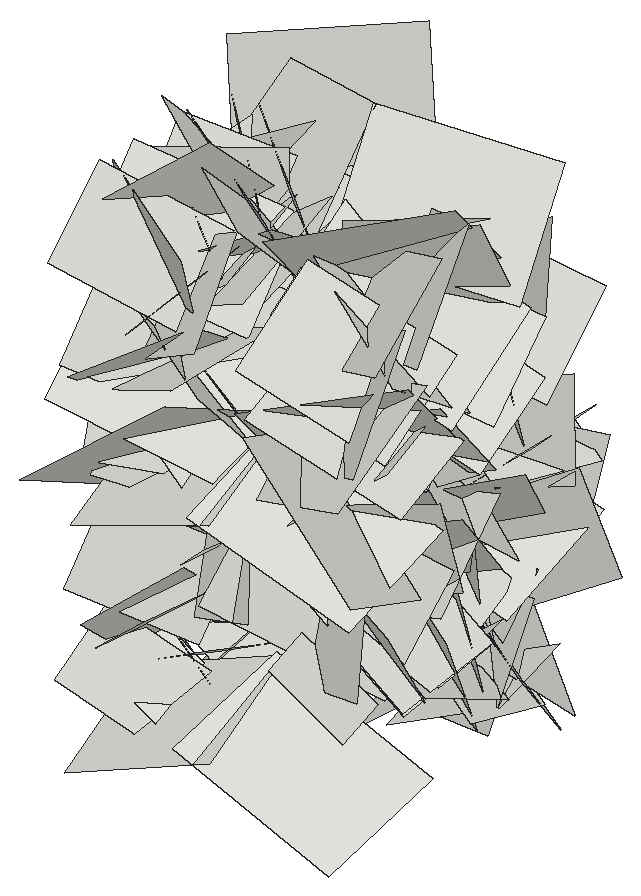
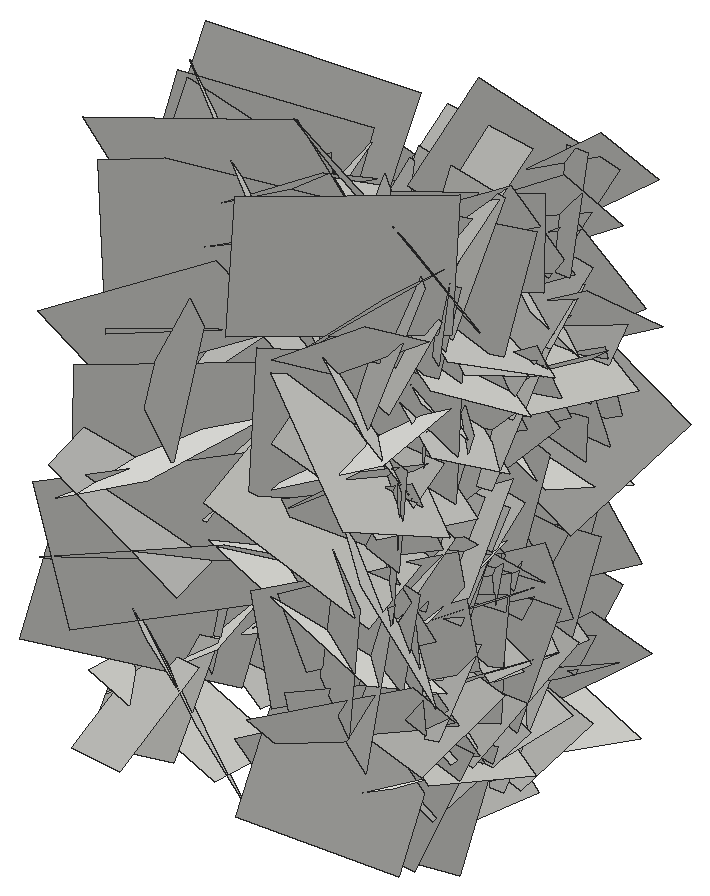
# SketchUp Ruby script. Lengths in inches.
U = 1.inch
M = Sketchup.active_model
def pt(a) = Geom::Point3d.new(a.map { |v| v * U })
def face(e, loops, mat)
  f = e.add_face(loops[0].map { |a| pt(a) })
  loops[1..].each { |l| e.add_face(l.map { |a| pt(a) }).erase! }
  f.material = f.back_material = mat if mat
  f
end
# faces: each face lists its corners as indices into pts; further lists are holes
def faces(e, pts, list, mat = nil) = list.each { |f| face(e, (f[0].is_a?(Array) ? f : [f]).map { |l| l.map { |i| pts[i] } }, mat) }
# xy, xz, yz: faces in a plane at the given z, y or x. An outline is a flat list of corners, or four numbers for a rectangle; further outlines are holes
def ring(l) = l.size == 4 ? [[l[0], l[1]], [l[2], l[1]], [l[2], l[3]], [l[0], l[3]]] : l.each_slice(2).to_a
def flat(e, list, mat, &to3) = list.each { |f| face(e, (f[0].is_a?(Array) ? f : [f]).map { |l| ring(l).map { |u, v| to3.(u, v) } }, mat) }
def xy(e, z, list, mat = nil) = flat(e, list, mat) { |x, y| [x, y, z] }
def xz(e, y, list, mat = nil) = flat(e, list, mat) { |x, z| [x, y, z] }
def yz(e, x, list, mat = nil) = flat(e, list, mat) { |y, z| [x, y, z] }
def lines(e, pts, list) = list.each { |a, b| e.add_line(pt(pts[a]), pt(pts[b])) }
# prism: a flat outline (further loops are holes) pulled along v
def prism(e, loops, v, mat = nil)
  f = face(e, loops, mat); d = Geom::Vector3d.new(v.map { |x| x * U })
  f.pushpull(f.normal.samedirection?(d) ? d.length : -d.length)
end
def box(e, o, s, mat = nil) = prism(e, [[o, [o[0] + s[0], o[1], o[2]], [o[0] + s[0], o[1] + s[1], o[2]], [o[0], o[1] + s[1], o[2]]]], [0, 0, s[2]], mat)
def at(x, y, z, deg = 0) = Geom::Transformation.translation(pt([x, y, z])) * Geom::Transformation.rotation(ORIGIN, Z_AXIS, deg.degrees)
def axes(o, x, y, z) = Geom::Transformation.new([*x, 0, *y, 0, *z, 0, *pt(o).to_a, 1])
def part(name) = M.definitions.add(name)
# library, detail: a bought-in or finely detailed component or shape, given as its bounding box
def library(name, o, s) = part(name).tap { |d| box(d.entities, o, s) }
def detail(e, o, s) = box(e.add_group.entities, o, s)
def put(e, d, t, mat = nil) = e.add_instance(d, t).tap { |i| i.material = mat if mat }
def group(e, t, mat = nil) = e.add_group.tap { |g| g.transformation = t; g.material = mat if mat }.entities
root = M.entities
c1 = part("Component\#6")
p = [[0.01,0,0],[0,3.24,4.54],[4.32,3.24,4.54],[4.33,0,0]]
faces(c1.entities,p,[[0,1,2,3]])
put(root,c1,axes([414.68,163.43,17.5],[0.07736,-0.30856,0.98844],[0.18729,0.98007,0.2929],[-1.08152,0.14765,0.12143]))
put(root,c1,axes([410.71,163.43,17.5],[-0.07736,-0.30856,0.98844],[-0.18729,0.98007,0.2929],[1.08152,0.14765,0.12143]))
put(root,c1,axes([410.71,155.625,2.89],[0.13104,0.56412,0.5606],[-0.11872,0.57403,-0.55293],[0.83462,-0.00692,-0.16667]))
put(root,c1,axes([410.71,168.54,15.47],[-0.051,0.16682,-0.79913],[0.09039,-0.79511,-0.17112],[0.86061,0.0934,-0.02938]))
put(root,c1,axes([414.68,164.44,22.83],[0.02931,-0.02413,-0.88007],[0.04764,-0.87932,0.02552],[-0.93201,-0.0457,-0.02637]))
put(root,c1,axes([410.71,159.9,13.67],[-0.02397,0.44215,0.82689],[-0.11898,0.8199,-0.44149],[0.98679,0.1096,-0.03314]))
put(root,c1,axes([410.71,159.79,6],[-0.13547,0.51146,0.93772],[-0.15367,0.92736,-0.52557],[1.12174,0.18881,0.04125]))
put(root,c1,axes([414.68,165.07,9.38],[-0.13081,0.27606,-0.70722],[0.08788,-0.70731,-0.29057],[-0.79993,-0.12284,0.08373]))
put(root,c1,axes([410.71,167.39,19.82],[0.12929,0.6108,0.35138],[0.02449,0.35295,-0.62154],[0.74654,-0.11736,-0.04046]))
put(root,c1,axes([410.71,155.24,20.59],[0.01301,0.69003,0.71111],[-0.211,0.69839,-0.67424],[1.02891,0.13449,-0.14726]))
put(root,c1,axes([410.71,164.66,7.18],[-0.03191,0.54978,-0.59147],[0.106,-0.58478,-0.54866],[0.84939,0.09364,0.04625]))
put(root,c1,axes([410.71,167.84,10.46],[-0.01526,0.23241,-0.73689],[0.14958,-0.72384,-0.23105],[0.80526,0.13886,0.02896]))
put(root,c1,axes([410.71,166.25,3.34],[0.10377,-0.78092,-0.09398],[-0.04515,-0.09983,0.78516],[0.83253,0.09192,0.05429]))
put(root,c1,axes([410.71,166.67,11.65],[0.03639,0.32382,0.70516],[0.0632,0.70266,-0.32558],[0.82009,-0.06852,-0.0062]))
put(root,c1,axes([414.68,164.7,6.68],[0.19863,-0.78204,0.62344],[0.03401,0.63866,0.7915],[-1.0596,-0.1261,0.14227]))
put(root,c1,axes([414.68,165.06,16.01],[0.24936,0.99659,0.4051],[0.07669,0.39908,-1.02378],[-1.13774,0.24532,0.01978]))
put(root,c1,axes([414.68,162.4,12.14],[-0.15913,-0.1111,0.71617],[0.10617,0.72117,0.13287],[-0.76084,0.12387,-0.13124]))
put(root,c1,axes([410.71,166.02,4.84],[-0.16866,0.71959,0.68076],[0.0323,0.69272,-0.72511],[1.04952,0.09433,0.13172]))
put(root,c1,axes([410.71,157.37,3.29],[0.12325,0.67494,0.21472],[0.06797,0.20667,-0.68436],[0.74769,-0.13004,0.02682]))
put(root,c1,axes([410.71,162.54,0.74],[-0.05881,-0.79857,0.25436],[0.14334,0.24305,0.79255],[0.87675,-0.0933,-0.11251]))
put(root,c1,axes([410.71,164.04,2.37],[-0.08884,-0.86849,0.07962],[0.14736,0.06566,0.86256],[0.91264,-0.09515,-0.13152]))
put(root,c1,axes([414.68,167.12,21.5],[-0.0656,0.35319,-0.61189],[-0.00255,-0.61434,-0.35436],[-0.7489,-0.02885,0.0548]))
put(root,c1,axes([414.68,165.55,15.88],[0.02597,-0.35934,-0.67832],[-0.02345,-0.67872,0.35875],[-0.81334,0.00809,-0.032]))
put(root,c1,axes([414.68,169.26,18.83],[-0.02849,-0.83115,-0.05333],[0.13283,-0.05679,0.82186],[-0.87278,0.01849,0.12683]))
put(root,c1,axes([410.71,168.08,9.41],[-0.11593,0.02752,-0.90523],[0.14705,-0.90054,-0.04413],[0.94866,0.14295,-0.10378]))
put(root,c1,axes([414.68,161.46,7.67],[-0.11157,-0.00104,0.59962],[-0.09459,0.60203,-0.01462],[-0.62852,-0.09042,-0.10424]))
put(root,c1,axes([414.68,169.83,13.22],[-0.13817,-0.64015,-0.16037],[0.03989,-0.17041,0.64965],[-0.69839,0.11692,0.06883]))
put(root,c1,axes([410.71,170.98,12.21],[-0.31631,-0.51758,-1.19288],[-0.16648,-1.20059,0.56021],[1.36826,-0.26573,-0.20761]))
put(root,c1,axes([414.68,164.04,15.7],[-0.03624,-0.6234,-0.24842],[-0.08,-0.24359,0.62167],[-0.70683,0.05954,-0.05762]))
put(root,c1,axes([414.68,160.57,3.12],[-0.03509,0.82869,0.13415],[0.15764,0.13792,-0.81528],[-0.87577,-0.00838,-0.15213]))
put(root,c1,axes([410.71,159.03,23.29],[-0.13252,0.38295,-0.87838],[0.10893,-0.87536,-0.39626],[1.00987,0.14467,-0.07253]))
put(root,c1,axes([414.68,166.8,6.58],[0.19077,-0.84984,-0.315],[-0.00737,-0.32244,0.86593],[-0.9607,-0.16629,-0.0692]))
put(root,c1,axes([410.71,166.22,16.78],[-0.0558,0.90138,-0.08554],[0.09664,-0.07998,-0.89882],[0.95488,0.06076,0.08597]))
put(root,c1,axes([414.68,159.32,12.84],[-0.06752,-0.16321,-0.59207],[-0.0871,-0.58763,0.17083],[-0.64514,0.09641,0.0389]))
put(root,c1,axes([410.71,167.39,3.05],[-0.22625,-1.02118,-0.283],[0.12014,-0.30902,1.02962],[1.11681,-0.17363,-0.16809]))
put(root,c1,axes([414.68,159.79,25.07],[0.1328,0.69586,-0.68383],[0.18687,-0.69425,-0.67416],[-1.01714,-0.03669,-0.21313]))
put(root,c1,axes([410.71,163.26,10.51],[0.09772,0.8385,-0.3881],[-0.10419,-0.37892,-0.842],[0.97385,-0.12468,-0.05114]))
put(root,c1,axes([414.68,160.97,6.7],[-0.04912,0.73058,0.10133],[0.09877,0.10652,-0.72536],[-0.77557,-0.03271,-0.0988]))
put(root,c1,axes([410.71,170.16,13.55],[-0.14984,-1.04824,-0.22204],[0.00627,-0.22472,1.05715],[1.13577,-0.13705,-0.03513]))
put(root,c1,axes([414.68,161.26,10.83],[0.08958,0.45503,-0.59155],[-0.06652,-0.58889,-0.46195],[-0.78829,0.10141,-0.02824]))
put(root,c1,axes([414.68,160.54,14.42],[0.065,-0.29459,-0.75204],[0.0763,-0.74921,0.29935],[-0.85274,-0.0895,-0.03054]))
put(root,c1,axes([414.68,160.65,18.69],[-0.1336,-0.1743,0.59472],[0.06624,0.60023,0.18916],[-0.65357,0.09646,-0.1024]))
put(root,c1,axes([414.68,159.61,12.59],[-0.0897,0.16152,-0.57424],[-0.01993,-0.58042,-0.16049],[-0.632,-0.00462,0.08656]))
put(root,c1,axes([410.71,169.09,13.37],[0.12805,-0.81492,0.2825],[-0.01832,0.28292,0.8235],[0.91406,0.11983,-0.02307]))
put(root,c1,axes([414.68,158.82,19.64],[-0.09205,0.73549,-0.019],[0.17536,0.00088,-0.72213],[-0.75991,-0.08889,-0.16434]))
put(root,c1,axes([410.71,166.72,20.27],[0.14718,0.45385,-0.66356],[0.05291,-0.67695,-0.45256],[0.85051,-0.03642,0.14299]))
put(root,c1,axes([410.71,158.84,13.7],[0.15038,-0.75335,0.50607],[-0.08727,0.49942,0.76653],[0.95804,0.16374,-0.00961]))
put(root,c1,axes([410.71,161.03,4.22],[0.00206,0.54706,-0.73945],[0.10036,-0.73565,-0.544],[0.96983,0.07497,0.05787]))
put(root,c1,axes([410.71,167.74,3.51],[-0.11337,-0.86322,0.3774],[0.28126,0.33685,0.84566],[0.95821,-0.201,-0.20357]))
put(root,c1,axes([410.71,165.75,-1.09],[-0.03685,-0.4153,0.96157],[-0.02645,0.96216,0.41465],[1.10996,0.00914,0.04181]))
put(root,c1,axes([410.71,165.51,17.74],[0.00528,-0.97827,-0.44464],[-0.11526,-0.44282,0.97306],[1.13321,-0.04048,0.10104]))
put(root,c1,axes([414.68,158.25,7.85],[-0.01053,0.60228,-0.51533],[0.19634,-0.49934,-0.58716],[-0.81696,-0.12777,-0.13447]))
put(root,c1,axes([414.68,167.39,12.19],[0.06725,0.11282,-0.6237],[-0.12717,-0.61335,-0.12315],[-0.65971,0.12973,-0.03984]))
put(root,c1,axes([414.68,164.71,11.17],[0.09162,-0.23701,0.75882],[0.09076,0.76162,0.22813],[-0.83777,0.05659,0.1077]))
put(root,c1,axes([410.71,164.72,6.23],[-0.02586,0.29335,1.1723],[-0.23754,1.1511,-0.29271],[1.25874,0.22326,-0.03115]))
put(root,c1,axes([414.68,159.82,10.86],[0.164,0.05549,-0.7166],[-0.119,-0.72215,-0.08015],[-0.75252,0.12629,-0.14349]))
put(root,c1,axes([410.71,167.01,8.33],[0.18631,0.3359,0.73427],[0.04897,0.74605,-0.35235],[0.8545,-0.11599,-0.1399]))
put(root,c1,axes([410.71,166.18,19.56],[-0.12535,0.0531,1.28965],[-0.2192,1.27754,-0.07157],[1.35051,0.21229,0.10808]))
put(root,c1,axes([410.71,168.14,0.12],[-0.06773,-0.63363,0.78179],[0.11595,0.77435,0.63654],[1.06038,-0.12515,-0.01967]))
put(root,c1,axes([410.71,169.19,10.7],[-0.0913,0.46499,-1.24639],[-0.29576,-1.22753,-0.43867],[1.37875,-0.23253,-0.17663]))
put(root,c1,axes([414.68,165.96,10.85],[0.09912,0.20412,-0.70693],[0.02587,-0.71308,-0.20267],[-0.77953,0.00229,-0.09661]))
put(root,c1,axes([414.68,161.25,17.66],[0.25985,0.898,-0.37026],[0.14737,-0.41038,-0.90325],[-1.01902,0.16964,-0.22504]))
put(root,c1,axes([414.68,162.79,15.86],[0.07285,0.46729,0.4905],[-0.02436,0.49435,-0.46773],[-0.71769,0.03066,0.06566]))
put(root,c1,axes([410.71,167.22,15.375],[-0.0235,-0.92066,-0.53568],[-0.01768,-0.53543,0.92093],[1.12894,-0.02755,0.00327]))
put(root,c1,axes([410.71,167.28,17.92],[-0.19972,-0.96368,-0.57877],[0.14667,-0.60226,0.95775],[1.18251,-0.08806,-0.21655]))
put(root,c1,axes([410.71,157.18,19.73],[-0.07599,0.81527,0.8297],[-0.084,0.82592,-0.8184],[1.23014,0.10676,-0.00463]))
put(root,c1,axes([410.71,167.18,1.59],[-0.07507,-1.0991,0.32301],[-0.05871,0.32653,1.09895],[1.2129,-0.05222,0.07319]))
put(root,c1,axes([410.71,168.87,14.79],[0.03205,0.06087,-1.12787],[-0.16204,-1.11767,-0.06442],[1.18627,-0.15431,0.02167]))
put(root,c1,axes([410.71,166.01,11.8],[0.21466,0.53877,-0.68228],[-0.03009,-0.69607,-0.55809],[0.92102,-0.14831,0.14079]))
put(root,c1,axes([410.71,163.57,3.71],[0.11292,-0.2033,0.99476],[-0.09749,0.99417,0.21302],[1.07181,0.11185,-0.08542]))
put(root,c1,axes([410.71,159.91,9.22],[-0.2022,-1.20502,0.50539],[-0.1049,0.52261,1.20871],[1.38114,-0.13672,0.1658]))
put(root,c1,axes([410.71,162.44,14.8125],[-0.22172,-1.13603,-0.19278],[0.19013,-0.22565,1.13507],[1.20652,-0.17321,-0.21429]))
put(root,c1,axes([410.71,160.62,5.12],[0.08568,1.04485,0.18773],[-0.09569,0.19436,-1.04286],[1.1212,-0.06325,-0.10335]))
put(root,c1,axes([414.68,162.91,7.6875],[0.03517,0.6334,0.29771],[0.1292,0.28826,-0.62688],[-0.73053,0.08147,-0.09654]))
put(root,c1,axes([410.71,163.93,5.47],[0.11462,-1.01834,-0.26907],[-0.10191,-0.2789,1.0169],[1.11183,0.07941,0.12095]))
put(root,c1,axes([410.71,156.14,6.5],[0.17845,0.35117,0.84391],[0.01887,0.85668,-0.36003],[0.96872,-0.08137,-0.14844]))
put(root,c1,axes([414.68,170.02,6.34],[0.13634,-0.30577,-0.6303],[0.02329,-0.63876,0.31436],[-0.74222,-0.07621,-0.10592]))
put(root,c1,axes([410.71,160.14,4.78],[0.03826,-0.47304,0.81506],[0.18962,0.80427,0.45886],[0.98077,-0.13704,-0.12051]))
put(root,c1,axes([410.71,166.625,12.7],[0.17127,1.04033,-0.10676],[-0.13463,-0.08771,-1.04688],[1.10034,-0.17266,-0.11147]))
put(root,c1,axes([410.71,168.99,0.33],[0.20008,-0.71049,0.66963],[-0.07161,0.67089,0.73087],[1.03242,0.18422,-0.07908]))
put(root,c1,axes([410.71,164.18,5.53],[0.00871,-1.21515,-0.1589],[-0.11926,-0.15898,1.20995],[1.29354,-0.00648,0.11262]))
put(root,c1,axes([414.68,159.77,13.93],[0.14822,0.47929,0.38572],[-0.01533,0.39801,-0.48932],[-0.65196,0.0996,0.0992]))
put(root,c1,axes([410.71,165.6875,8.33],[0.14254,-0.77018,0.64298],[0.05856,0.65343,0.77114],[1.06187,0.06735,-0.12884]))
put(root,c1,axes([410.71,164.53,2.65],[0.11418,0.95876,0.15487],[0.16789,0.13639,-0.95453],[1.01568,-0.13033,0.14037]))
put(root,c1,axes([414.68,155.94,6.59],[0.14653,0.65267,0.04592],[0.0729,0.03218,-0.6644],[-0.6897,0.14207,-0.06047]))
put(root,c1,axes([410.71,170.79,17.67],[0.07972,-0.69903,-0.88266],[-0.01234,-0.88506,0.69994],[1.19343,0.03754,0.0662]))
put(root,c1,axes([410.71,165.97,13.03],[0.11695,-0.23373,1.15092],[-0.10796,1.14973,0.24325],[1.24018,0.12213,-0.08736]))
put(root,c1,axes([414.68,164.09,3.1],[0.16189,-0.51758,0.36968],[0.06161,0.38995,0.52196],[-0.67139,-0.08902,0.13704]))
put(root,c1,axes([410.71,155.93,16.01],[0.06166,0.77521,1.08886],[-0.24821,1.07895,-0.75564],[1.39492,0.15772,-0.18259]))
put(root,c1,axes([410.71,163.21,2.24],[-0.08398,-0.53221,1.10764],[0.11648,1.10243,0.53756],[1.29738,-0.13342,0.02343]))
put(root,c1,axes([410.71,161.02,12.77],[0.04866,0.36936,-1.04237],[0.12613,-1.03886,-0.36288],[1.16543,0.09701,0.0828]))
put(root,c1,axes([410.71,162.03,18.62],[0.15865,-0.78055,-0.79386],[-0.03617,-0.80384,0.78393],[1.17956,0.08034,0.13081]))
put(root,c1,axes([410.71,161.03,16.77],[-0.02327,0.73455,-0.90907],[0.17416,-0.89826,-0.72978],[1.22657,0.14148,0.08637]))
put(root,c1,axes([410.71,163.86,1.73],[0.03729,0.66749,1.03354],[-0.00972,1.03407,-0.66752],[1.30413,-0.01138,-0.03452]))
put(root,c1,axes([410.71,162.85,15.75],[0.04254,-1.00522,0.67204],[0.02385,0.67292,1.00519],[1.28151,0.02084,-0.04102]))
put(root,c1,axes([410.71,163.36,23.49],[0.04873,0.57368,-1.00395],[0.12423,-1.00188,-0.56714],[1.21936,0.07915,0.09791]))
put(root,c1,axes([410.71,159.69,18.96],[0.02704,0.74145,1.09535],[-0.09362,1.09406,-0.73853],[1.39894,0.05888,-0.07059]))
put(root,c1,axes([410.71,166.4,18.65],[-0.092,-1.19571,-0.63762],[0.0325,-0.6405,1.19693],[1.43603,-0.06211,-0.06794]))
put(root,c1,axes([410.71,155.03,14.95],[-0.10989,1.07322,0.82249],[0.07177,0.82799,-1.07186],[1.43147,0.04087,0.11688]))
put(root,c1,axes([410.71,159.14,18.38],[0.07521,0.79304,-0.86536],[0.12573,-0.86735,-0.78513],[1.23784,0.03991,0.13233]))
put(root,c1,axes([410.71,168.375,23.9],[-0.0952,-0.72561,-1.04974],[0.29336,-1.03837,0.69407],[1.32049,0.17837,-0.22987]))
put(root,c1,axes([410.71,157.93,15.34],[0.27083,1.19165,0.15594],[-0.0802,0.17506,-1.21378],[1.27139,-0.2428,-0.10978]))
put(root,c1,axes([410.71,162.31,11.53],[0.17206,0.75955,-0.87532],[0.12131,-0.89005,-0.75111],[1.22246,-0.01858,0.19774]))
put(root,c1,axes([410.71,165.1,2.71],[-0.06092,-1.21711,0.58199],[0.18306,0.57109,1.21136],[1.41828,-0.12599,-0.13136]))
put(root,c1,axes([410.71,170.58,10.37],[0.24309,-1.14649,0.14454],[0.04952,0.15643,1.16674],[1.2239,0.22139,-0.07591]))
put(root,c1,axes([410.71,161.07,7.88],[0.0926,0.91308,0.78861],[0.24837,0.76278,-0.90913],[1.25453,-0.21841,0.12178]))
put(root,c1,axes([410.71,171.01,11.29],[0.23144,-0.15428,-1.27652],[-0.01824,-1.29503,0.15357],[1.36284,0.00887,0.21884]))
put(root,c1,axes([410.71,167.61,21.95],[0.32344,0.31012,-1.26322],[-0.1451,-1.28265,-0.34796],[1.37111,-0.2089,0.26116]))
put(root,c1,axes([410.71,161.91,24.73],[0.20116,0.87735,-0.9177],[0.06395,-0.93308,-0.87958],[1.34427,-0.0869,0.17917]))
put(root,c1,axes([410.71,161.24,11.55],[0.08722,-1.18104,-0.51149],[0.30261,-0.48302,1.16122],[1.33028,0.18731,-0.23062]))
put(root,c1,axes([410.71,160.65,1.35],[0.1594,-1.22011,-0.46707],[0.28659,-0.43091,1.2127],[1.35486,0.2347,-0.20157]))
put(root,c1,axes([410.71,170.67,8.29],[0.13658,-1.14766,-0.62909],[0.33753,-0.58565,1.13362],[1.34561,0.26339,-0.2205]))
put(root,c1,axes([410.71,161.87,9.58],[0.35888,-0.49511,-1.17449],[0.11741,-1.19919,0.53746],[1.34594,0.23663,0.26628]))
put(root,c1,axes([424.49,161.87,9.58],[-0.35888,-0.49511,-1.17449],[-0.11741,-1.19919,0.53746],[-1.34594,0.23663,0.26628]))
put(root,c1,axes([424.49,170.67,8.29],[-0.13658,-1.14766,-0.62909],[-0.33753,-0.58565,1.13362],[-1.34561,0.26339,-0.2205]))
put(root,c1,axes([424.49,160.65,1.35],[-0.1594,-1.22011,-0.46707],[-0.28659,-0.43091,1.2127],[-1.35486,0.2347,-0.20157]))
put(root,c1,axes([424.49,161.24,11.55],[-0.08722,-1.18104,-0.51149],[-0.30261,-0.48302,1.16122],[-1.33028,0.18731,-0.23062]))
put(root,c1,axes([424.49,161.91,24.73],[-0.20116,0.87735,-0.9177],[-0.06395,-0.93308,-0.87958],[-1.34427,-0.0869,0.17917]))
put(root,c1,axes([424.49,167.61,21.95],[-0.32344,0.31012,-1.26322],[0.1451,-1.28265,-0.34796],[-1.37111,-0.2089,0.26116]))
put(root,c1,axes([424.49,171.01,11.29],[-0.23144,-0.15428,-1.27652],[0.01824,-1.29503,0.15357],[-1.36284,0.00887,0.21884]))
put(root,c1,axes([424.49,161.07,7.88],[-0.0926,0.91308,0.78861],[-0.24837,0.76278,-0.90913],[-1.25453,-0.21841,0.12178]))
put(root,c1,axes([424.49,170.58,10.37],[-0.24309,-1.14649,0.14454],[-0.04952,0.15643,1.16674],[-1.2239,0.22139,-0.07591]))
put(root,c1,axes([424.49,165.1,2.71],[0.06092,-1.21711,0.58199],[-0.18306,0.57109,1.21136],[-1.41828,-0.12599,-0.13136]))
put(root,c1,axes([424.49,162.31,11.53],[-0.17206,0.75955,-0.87532],[-0.12131,-0.89005,-0.75111],[-1.22246,-0.01858,0.19774]))
put(root,c1,axes([424.49,157.93,15.34],[-0.27083,1.19165,0.15594],[0.0802,0.17506,-1.21378],[-1.27139,-0.2428,-0.10978]))
put(root,c1,axes([424.49,168.375,23.9],[0.0952,-0.72561,-1.04974],[-0.29336,-1.03837,0.69407],[-1.32049,0.17837,-0.22987]))
put(root,c1,axes([424.49,159.14,18.38],[-0.07521,0.79304,-0.86536],[-0.12573,-0.86735,-0.78513],[-1.23784,0.03991,0.13233]))
put(root,c1,axes([424.49,155.03,14.95],[0.10989,1.07322,0.82249],[-0.07177,0.82799,-1.07186],[-1.43147,0.04087,0.11688]))
put(root,c1,axes([424.49,166.4,18.65],[0.092,-1.19571,-0.63762],[-0.0325,-0.6405,1.19693],[-1.43603,-0.06211,-0.06794]))
put(root,c1,axes([424.49,159.69,18.96],[-0.02704,0.74145,1.09535],[0.09362,1.09406,-0.73853],[-1.39894,0.05888,-0.07059]))
put(root,c1,axes([424.49,163.36,23.49],[-0.04873,0.57368,-1.00395],[-0.12423,-1.00188,-0.56714],[-1.21936,0.07915,0.09791]))
put(root,c1,axes([424.49,162.85,15.75],[-0.04254,-1.00522,0.67204],[-0.02385,0.67292,1.00519],[-1.28151,0.02084,-0.04102]))
put(root,c1,axes([424.49,163.86,1.73],[-0.03729,0.66749,1.03354],[0.00972,1.03407,-0.66752],[-1.30413,-0.01138,-0.03452]))
put(root,c1,axes([424.49,161.03,16.77],[0.02327,0.73455,-0.90907],[-0.17416,-0.89826,-0.72978],[-1.22657,0.14148,0.08637]))
put(root,c1,axes([424.49,162.03,18.62],[-0.15865,-0.78055,-0.79386],[0.03617,-0.80384,0.78393],[-1.17956,0.08034,0.13081]))
put(root,c1,axes([424.49,161.02,12.77],[-0.04866,0.36936,-1.04237],[-0.12613,-1.03886,-0.36288],[-1.16543,0.09701,0.0828]))
put(root,c1,axes([424.49,163.21,2.24],[0.08398,-0.53221,1.10764],[-0.11648,1.10243,0.53756],[-1.29738,-0.13342,0.02343]))
put(root,c1,axes([424.49,155.93,16.01],[-0.06166,0.77521,1.08886],[0.24821,1.07895,-0.75564],[-1.39492,0.15772,-0.18259]))
put(root,c1,axes([420.52,164.09,3.1],[-0.16189,-0.51758,0.36968],[-0.06161,0.38995,0.52196],[0.67139,-0.08902,0.13704]))
put(root,c1,axes([424.49,165.97,13.03],[-0.11695,-0.23373,1.15092],[0.10796,1.14973,0.24325],[-1.24018,0.12213,-0.08736]))
put(root,c1,axes([424.49,170.79,17.67],[-0.07972,-0.69903,-0.88266],[0.01234,-0.88506,0.69994],[-1.19343,0.03754,0.0662]))
put(root,c1,axes([420.52,155.94,6.59],[-0.14653,0.65267,0.04592],[-0.0729,0.03218,-0.6644],[0.6897,0.14207,-0.06047]))
put(root,c1,axes([424.49,164.53,2.65],[-0.11418,0.95876,0.15487],[-0.16789,0.13639,-0.95453],[-1.01568,-0.13033,0.14037]))
put(root,c1,axes([424.49,165.6875,8.33],[-0.14254,-0.77018,0.64298],[-0.05856,0.65343,0.77114],[-1.06187,0.06735,-0.12884]))
put(root,c1,axes([420.52,159.77,13.93],[-0.14822,0.47929,0.38572],[0.01533,0.39801,-0.48932],[0.65196,0.0996,0.0992]))
put(root,c1,axes([424.49,164.18,5.53],[-0.00871,-1.21515,-0.1589],[0.11926,-0.15898,1.20995],[-1.29354,-0.00648,0.11262]))
put(root,c1,axes([424.49,168.99,0.33],[-0.20008,-0.71049,0.66963],[0.07161,0.67089,0.73087],[-1.03242,0.18422,-0.07908]))
put(root,c1,axes([424.49,166.625,12.7],[-0.17127,1.04033,-0.10676],[0.13463,-0.08771,-1.04688],[-1.10034,-0.17266,-0.11147]))
put(root,c1,axes([424.49,160.14,4.78],[-0.03826,-0.47304,0.81506],[-0.18962,0.80427,0.45886],[-0.98077,-0.13704,-0.12051]))
put(root,c1,axes([420.52,170.02,6.34],[-0.13634,-0.30577,-0.6303],[-0.02329,-0.63876,0.31436],[0.74222,-0.07621,-0.10592]))
put(root,c1,axes([424.49,156.14,6.5],[-0.17845,0.35117,0.84391],[-0.01887,0.85668,-0.36003],[-0.96872,-0.08137,-0.14844]))
put(root,c1,axes([424.49,163.93,5.47],[-0.11462,-1.01834,-0.26907],[0.10191,-0.2789,1.0169],[-1.11183,0.07941,0.12095]))
put(root,c1,axes([420.52,162.91,7.6875],[-0.03517,0.6334,0.29771],[-0.1292,0.28826,-0.62688],[0.73053,0.08147,-0.09654]))
put(root,c1,axes([424.49,160.62,5.12],[-0.08568,1.04485,0.18773],[0.09569,0.19436,-1.04286],[-1.1212,-0.06325,-0.10335]))
put(root,c1,axes([424.49,162.44,14.8125],[0.22172,-1.13603,-0.19278],[-0.19013,-0.22565,1.13507],[-1.20652,-0.17321,-0.21429]))
put(root,c1,axes([424.49,159.91,9.22],[0.2022,-1.20502,0.50539],[0.1049,0.52261,1.20871],[-1.38114,-0.13672,0.1658]))
put(root,c1,axes([424.49,163.57,3.71],[-0.11292,-0.2033,0.99476],[0.09749,0.99417,0.21302],[-1.07181,0.11185,-0.08542]))
put(root,c1,axes([424.49,166.01,11.8],[-0.21466,0.53877,-0.68228],[0.03009,-0.69607,-0.55809],[-0.92102,-0.14831,0.14079]))
put(root,c1,axes([424.49,168.87,14.79],[-0.03205,0.06087,-1.12787],[0.16204,-1.11767,-0.06442],[-1.18627,-0.15431,0.02167]))
put(root,c1,axes([424.49,167.18,1.59],[0.07507,-1.0991,0.32301],[0.05871,0.32653,1.09895],[-1.2129,-0.05222,0.07319]))
put(root,c1,axes([424.49,157.18,19.73],[0.07599,0.81527,0.8297],[0.084,0.82592,-0.8184],[-1.23014,0.10676,-0.00463]))
put(root,c1,axes([424.49,167.28,17.92],[0.19972,-0.96368,-0.57877],[-0.14667,-0.60226,0.95775],[-1.18251,-0.08806,-0.21655]))
put(root,c1,axes([424.49,167.22,15.375],[0.0235,-0.92066,-0.53568],[0.01768,-0.53543,0.92093],[-1.12894,-0.02755,0.00327]))
put(root,c1,axes([420.52,162.79,15.86],[-0.07285,0.46729,0.4905],[0.02436,0.49435,-0.46773],[0.71769,0.03066,0.06566]))
put(root,c1,axes([420.52,161.25,17.66],[-0.25985,0.898,-0.37026],[-0.14737,-0.41038,-0.90325],[1.01902,0.16964,-0.22504]))
put(root,c1,axes([420.52,165.96,10.85],[-0.09912,0.20412,-0.70693],[-0.02587,-0.71308,-0.20267],[0.77953,0.00229,-0.09661]))
put(root,c1,axes([424.49,169.19,10.7],[0.0913,0.46499,-1.24639],[0.29576,-1.22753,-0.43867],[-1.37875,-0.23253,-0.17663]))
put(root,c1,axes([424.49,168.14,0.12],[0.06773,-0.63363,0.78179],[-0.11595,0.77435,0.63654],[-1.06038,-0.12515,-0.01967]))
